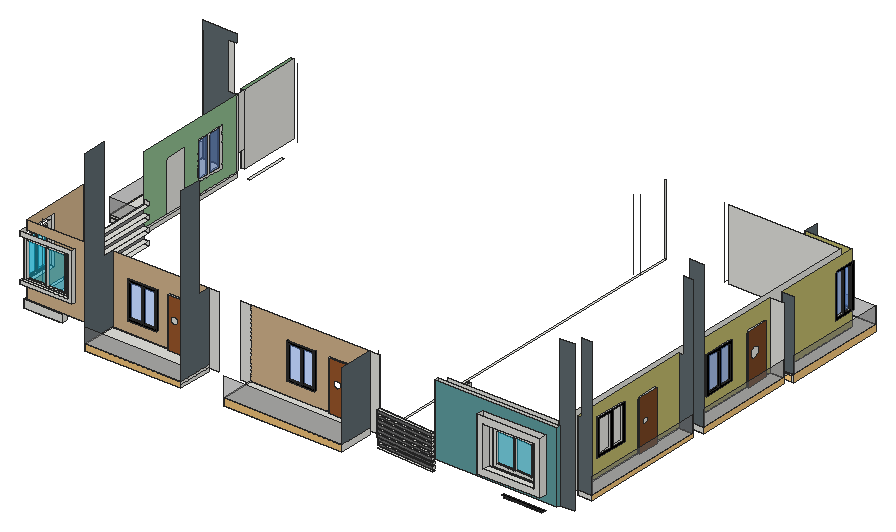
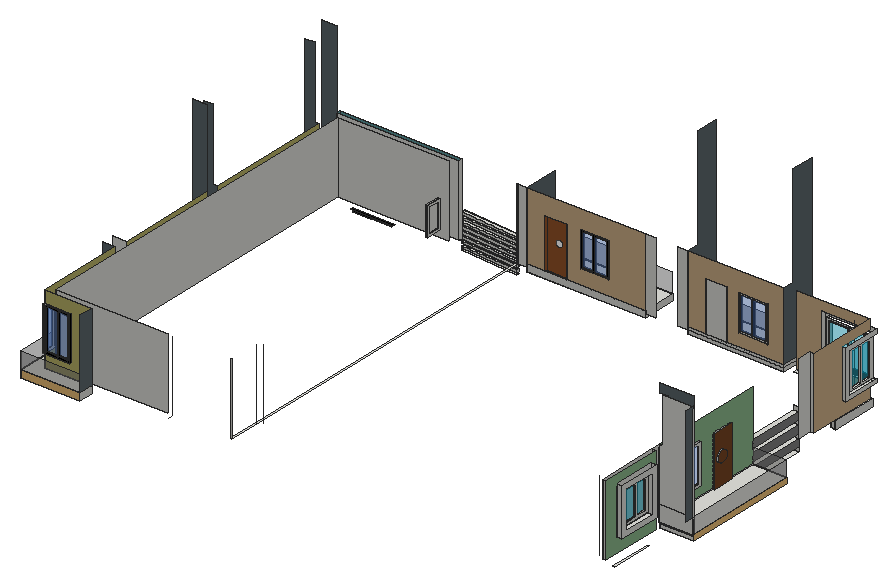
# SketchUp Ruby script. Lengths in inches.
U = 1.inch
M = Sketchup.active_model
def pt(a) = Geom::Point3d.new(a.map { |v| v * U })
def face(e, loops, mat)
  f = e.add_face(loops[0].map { |a| pt(a) })
  loops[1..].each { |l| e.add_face(l.map { |a| pt(a) }).erase! }
  f.material = f.back_material = mat if mat
  f
end
# faces: each face lists its corners as indices into pts; further lists are holes
def faces(e, pts, list, mat = nil) = list.each { |f| face(e, (f[0].is_a?(Array) ? f : [f]).map { |l| l.map { |i| pts[i] } }, mat) }
# xy, xz, yz: faces in a plane at the given z, y or x. An outline is a flat list of corners, or four numbers for a rectangle; further outlines are holes
def ring(l) = l.size == 4 ? [[l[0], l[1]], [l[2], l[1]], [l[2], l[3]], [l[0], l[3]]] : l.each_slice(2).to_a
def flat(e, list, mat, &to3) = list.each { |f| face(e, (f[0].is_a?(Array) ? f : [f]).map { |l| ring(l).map { |u, v| to3.(u, v) } }, mat) }
def xy(e, z, list, mat = nil) = flat(e, list, mat) { |x, y| [x, y, z] }
def xz(e, y, list, mat = nil) = flat(e, list, mat) { |x, z| [x, y, z] }
def yz(e, x, list, mat = nil) = flat(e, list, mat) { |y, z| [x, y, z] }
def lines(e, pts, list) = list.each { |a, b| e.add_line(pt(pts[a]), pt(pts[b])) }
# prism: a flat outline (further loops are holes) pulled along v
def prism(e, loops, v, mat = nil)
  f = face(e, loops, mat); d = Geom::Vector3d.new(v.map { |x| x * U })
  f.pushpull(f.normal.samedirection?(d) ? d.length : -d.length)
end
def box(e, o, s, mat = nil) = prism(e, [[o, [o[0] + s[0], o[1], o[2]], [o[0] + s[0], o[1] + s[1], o[2]], [o[0], o[1] + s[1], o[2]]]], [0, 0, s[2]], mat)
def at(x, y, z, deg = 0) = Geom::Transformation.translation(pt([x, y, z])) * Geom::Transformation.rotation(ORIGIN, Z_AXIS, deg.degrees)
def axes(o, x, y, z) = Geom::Transformation.new([*x, 0, *y, 0, *z, 0, *pt(o).to_a, 1])
def part(name) = M.definitions.add(name)
# library, detail: a bought-in or finely detailed component or shape, given as its bounding box
def library(name, o, s) = part(name).tap { |d| box(d.entities, o, s) }
def detail(e, o, s) = box(e.add_group.entities, o, s)
def put(e, d, t, mat = nil) = e.add_instance(d, t).tap { |i| i.material = mat if mat }
def group(e, t, mat = nil) = e.add_group.tap { |g| g.transformation = t; g.material = mat if mat }.entities
root = M.entities
M.materials.add("[0035_Tan]").color = [210, 180, 140]
M.materials.add("[0057_DarkKhaki]").color = [189, 183, 107]
M.materials.add("[0072_DarkSeaGreen]").color = [143, 188, 143]
M.materials.add("[0081_CadetBlue]").color = [95, 158, 160]
M.materials.add("[0133_Gray]").color = [128, 128, 128]
M.materials.add("[0134_DimGray]").color = [105, 105, 105]
M.materials.add("[0137_Black]").color = [0, 0, 0]
M.materials.add("[Formica Speckled Grey]").color = [94, 105, 111]
M.materials.add("[Translucent Glass Blue]").color = [100, 149, 237]
M.materials["[Translucent Glass Blue]"].alpha = 0.5
M.materials.add("[Translucent Glass Gray]").color = [128, 128, 128]
M.materials["[Translucent Glass Gray]"].alpha = 0.5
M.materials.add("[Translucent Glass Tinted]").color = [8, 201, 241]
M.materials["[Translucent Glass Tinted]"].alpha = 0.48
M.materials.add("[Wood Cherry Original]").color = [152, 86, 42]
M.materials.add("[Wood OSB]").color = [240, 195, 122]
M.materials.add("[Wood Veneer 01]").color = [120, 70, 37]
xy(root,471.13,[[972.47,731.11,975.47,770.48]])
xy(root,471.13,[[931.65,770.48,972.47,773.48],[972.47,770.48,975.47,773.48]],"[0137_Black]")
xy(root,471.63,[[80.8125,615.71,83.8125,687.27]])
xy(root,472.53,[[912.27,155.58,914.48,158.58]])
xy(root,472.53,[[880.02,155.58,912.27,158.58],[914.48,155.58,944.52,158.58]],"[0137_Black]")
xy(root,472.62,[[83.8125,295.24,92.8125,392.06]])
xy(root,474.43,[[766.19,148.96,766.41,152.52,668.06,158.52,667.84,154.96]])
xy(root,474.85,[[86.8125,155.58,108.25,158.58],[109.36,155.58,129.6875,158.58],[86.8125,158.58,108.25,158.77],[109.36,158.58,129.6875,158.77],[80.8125,161.58,83.8125,184.96],
  [80.8125,186.77,83.8125,211.96]])
xy(root,475.53,[[877.02,155.58,947.52,158.58]],"[0137_Black]")
xy(root,477.48,[[766.19,148.96,667.84,154.96,668.06,158.52,766.41,152.52]])
xy(root,477.85,[[80.8125,155.58,83.8125,158.77],[83.8125,155.58,132.6875,158.58],[83.8125,158.58,132.6875,158.77],[80.8125,158.77,83.8125,214.96]])
xy(root,479.56,[[74.8125,149.58,74.8125,227.52,83.8125,227.52,83.8125,158.58,140.48,158.58,140.48,149.58]])
xy(root,480.06,[[83.8125,295.24,92.8125,392.06]])
xy(root,481.68,[[766.19,148.96,766.41,152.52,668.06,158.52,667.84,154.96]])
xy(root,482.83,[[975.47,621.6875,975.47,770.48,896.3125,770.48,896.3125,794.48,996.47,794.48,996.47,621.6875]],"[Wood OSB]")
xy(root,484.73,[[766.19,148.96,667.84,154.96,668.06,158.52,766.41,152.52]])
xy(root,485.43,[[450.92,100.8,651.23,158.58]],"[Wood OSB]")
xy(root,486.18,[[217.79,100.8,379.72,158.58],[26.03,392.06,83.8125,587.65]],"[Wood OSB]")
xy(root,488.93,[[766.19,148.96,766.41,152.52,668.06,158.52,667.84,154.96]])
xy(root,489.56,[[972.47,431.23,996.47,600.85]],"[Wood OSB]")
xy(root,491.98,[[766.05,146.53,667.69,152.53,668.06,158.52,766.41,152.52]])
xy(root,492.18,[[74.8125,149.58,140.48,149.58,140.48,152.58,77.8125,152.58,77.8125,227.52,74.8125,227.52],[77.8125,152.58,83.8125,158.58],[83.8125,152.58,140.48,158.58],[140.48,152.58,200.97,158.58],[765.79,152.58,766.41,158.58],
  [766.41,152.58,972.47,158.58],[77.8125,158.58,83.8125,227.52],[666.68,158.58,668.06,709.05],[77.8125,227.52,83.8125,271.7],[77.8125,604.3125,83.8125,709.05],
  [666.68,709.05,668.06,761.48]])
xy(root,492.18,[[972.47,194.93,996.47,408.53]],"[Wood OSB]")
xy(root,492.56,[[83.8125,295.24,92.8125,392.06]])
xy(root,494.83,[[975.47,621.6875,996.47,621.6875,996.47,794.48,896.3125,794.48,896.3125,770.48,975.47,770.48]])
xy(root,496.06,[[26.03,392.06,83.8125,392.06,83.8125,440.49,80.8125,440.49,80.8125,476.49,83.8125,476.49,83.8125,587.65,26.03,587.65],[80.8125,440.49,83.8125,476.49],[26.03,587.65,83.8125,589.72]])
xy(root,496.18,[[766.05,146.53,766.41,152.52,668.06,158.52,667.69,152.53]])
xy(root,496.47,[[217.79,100.8,379.72,100.8,379.72,158.58,349.74,158.58,349.74,155.58,313.74,155.58,313.74,158.58,217.79,158.58],[450.92,100.8,651.23,100.8,651.23,158.58,620.77,158.58,620.77,155.58,584.77,155.58,584.77,158.58,450.92,158.58],[313.74,155.58,349.74,158.58],[584.77,155.58,620.77,158.58]])
xy(root,498.56,[[972.47,431.23,996.47,431.23,996.47,600.85,972.47,600.85,972.47,588.41,975.47,588.41,975.47,552.41,972.47,552.41],[972.47,552.41,975.47,588.41]])
xy(root,499.19,[[972.47,194.93,996.47,194.93,996.47,408.53,972.47,408.53,972.47,358.375,975.47,358.375,975.47,322.375,972.47,322.375],[972.47,322.375,975.47,358.375]])
xy(root,499.23,[[766.05,146.53,667.69,152.53,668.06,158.52,766.41,152.52]])
xy(root,500,[[83.8125,295.24,92.8125,392.06]])
xy(root,503.43,[[766.05,146.53,766.41,152.52,668.06,158.52,667.69,152.53]])
xy(root,503.75,[[846.5,140.58,952.45,152.58]])
xy(root,506.48,[[766.05,146.53,667.69,152.53,668.06,158.52,766.41,152.52]])
xy(root,510.68,[[766.05,146.53,766.41,152.52,668.06,158.52,667.69,152.53]])
xy(root,512.5,[[83.8125,295.24,92.8125,392.06]])
xy(root,513.73,[[766.05,146.53,667.69,152.53,668.06,158.52,766.41,152.52]])
xy(root,514.41,[[857.16,140.58,941.79,152.58]])
xy(root,514.48,[[80.8125,505.73,83.8125,555.41]])
xy(root,515.54,[[71.8125,146.58,71.8125,211.02,77.8125,211.02,77.8125,152.58,159.375,152.58,159.375,146.58]])
xy(root,517.48,[[80.8125,508.73,83.8125,527.36],[80.8125,530.57,83.8125,552.41]])
xy(root,517.58,[[245.3125,155.58,294.5,158.58]])
xy(root,517.93,[[766.05,146.53,766.41,152.52,668.06,158.52,667.69,152.53]])
xy(root,518.04,[[68.8125,613.85,77.8125,685.91]])
xy(root,518.4,[[866.65,149.58,936.8125,152.58]])
xy(root,518.53,[[930.09,770.48,972.47,773.48]])
xy(root,518.59,[[972.47,735.61,975.47,770.48],[972.47,770.48,975.47,773.48]])
xy(root,519.94,[[83.8125,295.24,92.8125,392.06]])
xy(root,520.39,[[514.1,155.58,560.92,158.58]],"[0137_Black]")
xy(root,520.58,[[248.3125,155.58,269.91,158.58],[272.57,155.58,291.5,158.58]],"[0137_Black]")
xy(root,520.98,[[766.05,146.53,667.69,152.53,668.06,158.52,766.41,152.52]])
xy(root,521.53,[[933.09,770.48,948.82,773.48],[951.28,770.48,969.47,773.48]],"[0137_Black]")
xy(root,521.54,[[71.8125,146.58,151.54,146.58,151.54,152.58,77.8125,152.58,77.8125,203.77,71.8125,203.77]])
xy(root,521.59,[[972.47,738.61,975.47,753.05],[972.47,755.68,975.47,767.48]],"[0137_Black]")
xy(root,522.6,[[74.8125,149.58,147.9375,152.58],[74.8125,152.58,77.8125,197.89]])
xy(root,523.39,[[517.1,155.58,537.51,158.58],[540.34,155.58,557.92,158.58]],"[0137_Black]")
xy(root,523.48,[[972.47,464.5,975.47,516.9375]])
xy(root,523.95,[[872.2,149.58,901.73,152.58],[904.37,149.58,931.26,152.58]])
xy(root,525.18,[[766.05,146.53,766.41,152.52,668.06,158.52,667.69,152.53]])
xy(root,525.6,[[80.8125,149.58,112.875,152.58],[114.7,149.58,144.9375,152.58],[74.8125,155.58,77.8125,172.52],[74.8125,175.24,77.8125,194.89]])
xy(root,525.84,[[68.8125,621.65,77.8125,678.11]])
xy(root,526.48,[[972.47,467.5,975.47,490.72],[972.47,493.16,975.47,513.9375]],"[0137_Black]")
xy(root,527.53,[[763.41,201.89,766.41,227.45]])
xy(root,528.23,[[766.05,146.53,667.69,152.53,668.06,158.52,766.41,152.52]])
xy(root,529.02,[[74.8125,624.83,77.8125,674.93]])
xy(root,530.53,[[763.41,204.89,766.41,224.45]])
xy(root,531.54,[[972.47,234.17,975.47,290.11]])
xy(root,532.35,[[74.8125,628.16,77.8125,647],[74.8125,649.88,77.8125,671.6]])
xy(root,532.43,[[766.05,146.53,766.41,152.52,668.06,158.52,667.69,152.53],[83.8125,295.24,92.8125,392.06]])
xy(root,572.16,[[763.41,204.89,766.41,224.45]])
xy(root,575.16,[[763.41,201.89,766.41,227.45]])
xz(root,100.8,[[217.79,496.47,379.72,522.05],[450.92,496.47,651.23,529.78]],"[Translucent Glass Gray]")
xz(root,100.8,[[450.92,485.43,651.23,496.47],[217.79,486.18,379.72,496.47]],"[Wood OSB]")
xz(root,140.58,[[[846.5,503.75,952.45,593.76],[857.16,514.41,941.79,583.1]]])
xz(root,146.58,[[71.8125,515.54,159.375,515.54,159.375,596.48,71.8125,596.48,71.8125,588.98,151.54,588.98,151.54,521.54,71.8125,521.54]])
xz(root,149.58,[[74.8125,479.56,140.48,492.18],[[866.65,518.4,936.8125,579.13],[872.2,523.95,901.73,573.58],[904.37,523.95,931.26,573.58]],[[74.8125,522.6,147.9375,586.79],[80.8125,525.6,112.875,583.79],[114.7,525.6,144.9375,583.79]]])
xz(root,152.58,[[[846.5,503.75,952.45,593.76],[857.16,514.41,941.79,583.1]],[[857.16,514.41,941.79,583.1],[866.65,518.4,936.8125,579.13]],[[866.65,518.4,936.8125,579.13],[872.2,523.95,901.73,573.58],[904.37,523.95,931.26,573.58]],[77.8125,521.54,151.54,521.54,151.54,588.98,77.8125,588.98,77.8125,586.79,147.9375,586.79,147.9375,522.6,77.8125,522.6]])
xz(root,152.58,[[77.8125,492.18,200.97,492.18,200.97,612.18,77.8125,612.18,77.8125,596.48,159.375,596.48,159.375,515.54,77.8125,515.54]],"[0035_Tan]")
xz(root,152.58,[[[766.41,492.18,972.47,612.18],[846.5,503.75,952.45,593.76]]],"[0081_CadetBlue]")
xz(root,152.58,[[872.2,523.95,901.73,573.58],[904.37,523.95,931.26,573.58],[80.8125,525.6,112.875,583.79],[114.7,525.6,144.9375,583.79]],"[Translucent Glass Tinted]")
xz(root,155.58,[[74.8125,525.6,77.8125,583.79]])
xz(root,155.58,[[[245.3125,517.58,294.5,579.7],[248.3125,520.58,269.91,576.7],[272.57,520.58,291.5,576.7]],[[514.1,520.39,560.92,580.89],[517.1,523.39,537.51,577.89],[540.34,523.39,557.92,577.89]]],"[0137_Black]")
xz(root,155.58,[[[313.74,496.47,349.74,580.47],[323.72,538.36,322.125,538.6875,320.67,539.43,319.45,540.51,318.5625,541.88,318.05,543.43,317.96,545.06,318.29,546.65,319.03,548.11,320.12,549.33,321.48,550.22,323.03,550.73,324.66,550.82,326.26,550.49,327.72,549.75,328.93,548.66,329.82,547.3,330.33,545.75,330.43,544.12,330.09,542.52,329.36,541.07,328.27,539.85,326.9,538.96,325.35,538.45]],[[584.77,496.47,620.77,580.47],[599.13,537.91,597.53,538.12,596.04,538.73,594.75,539.72,593.77,541,593.15,542.49,592.94,544.09,593.15,545.69,593.77,547.1875,594.75,548.47,596.04,549.45,597.53,550.07,599.13,550.28,600.73,550.07,602.22,549.45,603.5,548.47,604.49,547.1875,605.11,545.69,605.32,544.09,605.11,542.49,604.49,541,603.5,539.72,602.22,538.73,600.73,538.12]]],"[Wood Cherry Original]")
xz(root,158.58,[[83.8125,479.56,140.48,492.18],[450.92,485.43,651.23,496.47],[217.79,486.18,379.72,492.18],[217.79,492.18,379.72,496.47],[379.72,492.18,396.54,612.18],
  [434.03,492.18,450.85,612.18],[651.23,492.18,666.68,612.18],[666.68,492.18,668.06,612.18],[766.41,492.18,972.47,612.18],[313.74,496.47,349.74,580.47],
  [[245.3125,517.58,294.5,579.7],[248.3125,520.58,269.91,576.7],[272.57,520.58,291.5,576.7]]])
xz(root,158.58,[[[450.85,492.18,450.92,492.18,450.92,496.47,584.77,496.47,584.77,580.47,620.77,580.47,620.77,496.47,651.23,496.47,651.23,612.18,450.85,612.18],[514.1,520.39,560.92,580.89]],[[217.79,496.47,313.74,496.47,313.74,580.47,349.74,580.47,349.74,496.47,379.72,496.47,379.72,612.18,217.79,612.18],[245.3125,517.58,294.5,579.7]]],"[0035_Tan]")
xz(root,158.58,[[972.47,492.18,996.47,744.18]],"[Formica Speckled Grey]")
xz(root,158.58,[[248.3125,520.58,269.91,576.7],[272.57,520.58,291.5,576.7],[517.1,523.39,537.51,577.89],[540.34,523.39,557.92,577.89]],"[Translucent Glass Blue]")
xz(root,167.58,[[775.41,492.18,963.47,612.18]])
xz(root,172.52,[[74.8125,525.6,77.8125,583.79]])
xz(root,175.24,[[74.8125,525.6,77.8125,583.79]])
xz(root,194.89,[[74.8125,525.6,77.8125,583.79]])
xz(root,194.93,[[972.47,492.18,996.47,499.19]])
xz(root,194.93,[[972.47,499.19,972.47,612.18,980.72,612.18,980.72,732.18,996.47,732.18,996.47,499.19]],"[Formica Speckled Grey]")
xz(root,197.89,[[74.8125,522.6,77.8125,586.79]])
xz(root,201.89,[[763.41,527.53,766.41,575.16]])
xz(root,203.77,[[71.8125,521.36,77.8125,521.54],[71.8125,521.54,77.8125,588.98]])
xz(root,204.89,[[763.41,530.53,766.41,572.16]])
xz(root,211.02,[[71.8125,515.54,77.8125,596.48]])
xz(root,224.45,[[763.41,530.53,766.41,572.16]])
xz(root,227.45,[[763.41,527.53,766.41,575.16]])
xz(root,227.52,[[74.8125,479.56,77.8125,492.18],[77.8125,479.56,83.8125,492.18]])
xz(root,234.17,[[972.47,531.54,975.47,592.54]],"[0137_Black]")
xz(root,271.7,[[77.8125,492.18,83.8125,612.18]])
xz(root,290.11,[[972.47,531.54,975.47,592.54]],"[0137_Black]")
xz(root,295.24,[[83.8125,472.62,92.8125,480.06],[83.8125,492.56,92.8125,500],[83.8125,512.5,92.8125,519.94],[83.8125,532.43,92.8125,539.88]])
xz(root,322.375,[[972.47,499.19,975.47,583.19]],"[Wood Veneer 01]")
xz(root,358.375,[[972.47,499.19,975.47,583.19]],"[Wood Veneer 01]")
xz(root,392.06,[[83.8125,472.62,92.8125,480.06],[26.03,486.18,83.8125,492.18],[26.03,492.18,83.8125,492.56],[26.03,492.56,83.8125,496.06],[83.8125,492.56,92.8125,500],
  [83.8125,512.5,92.8125,519.94],[83.8125,532.43,92.8125,539.88]])
xz(root,392.06,[[26.03,496.06,83.8125,522.85]],"[Translucent Glass Gray]")
xz(root,408.53,[[972.47,492.18,996.47,499.19]])
xz(root,408.53,[[972.47,499.19,996.47,499.19,996.47,732.18,981.03,732.18,981.03,612.18,972.47,612.18]],"[Formica Speckled Grey]")
xz(root,431.23,[[972.47,489.56,996.47,498.56]])
xz(root,431.23,[[972.47,498.56,996.47,744.18]],"[Formica Speckled Grey]")
xz(root,440.49,[[80.8125,496.06,83.8125,580.06]],"[Wood Veneer 01]")
xz(root,464.5,[[972.47,523.48,975.47,585.79]],"[0137_Black]")
xz(root,467.5,[[972.47,526.48,975.47,582.79]],"[0137_Black]")
xz(root,476.49,[[80.8125,496.06,83.8125,580.06]],"[Wood Veneer 01]")
xz(root,490.72,[[972.47,526.48,975.47,582.79]],"[0137_Black]")
xz(root,493.16,[[972.47,526.48,975.47,582.79]],"[0137_Black]")
xz(root,505.73,[[80.8125,514.48,83.8125,580.48]])
xz(root,508.73,[[80.8125,517.48,83.8125,577.48]])
xz(root,513.9375,[[972.47,526.48,975.47,582.79]],"[0137_Black]")
xz(root,516.9375,[[972.47,523.48,975.47,585.79]],"[0137_Black]")
xz(root,527.36,[[80.8125,517.48,83.8125,577.48]])
xz(root,530.57,[[80.8125,517.48,83.8125,577.48]])
xz(root,552.41,[[80.8125,517.48,83.8125,577.48]])
xz(root,552.41,[[972.47,498.56,975.47,582.56]],"[Wood Veneer 01]")
xz(root,555.41,[[80.8125,514.48,83.8125,580.48]])
xz(root,587.65,[[26.03,486.18,83.8125,492.18],[26.03,492.18,83.8125,496.06]])
xz(root,587.65,[[26.03,496.06,83.8125,496.06,83.8125,612.18,68.8125,612.18,68.8125,689.85,83.8125,689.85,83.8125,704.68,26.03,704.68]],"[Formica Speckled Grey]")
xz(root,588.41,[[972.47,498.56,975.47,582.56]],"[Wood Veneer 01]")
xz(root,589.72,[[26.03,496.06,83.8125,522.6],[26.03,522.6,83.8125,522.6,83.8125,612.18,77.8125,612.18,77.8125,689.85,26.03,689.85]])
xz(root,600.85,[[972.47,489.56,996.47,498.56],[972.47,498.56,996.47,612.18]])
xz(root,604.3125,[[77.8125,492.18,83.8125,522.6],[77.8125,522.6,83.8125,612.18]])
xz(root,613.85,[[68.8125,518.04,77.8125,597.29]])
xz(root,621.65,[[68.8125,525.84,77.8125,589.49]])
xz(root,621.6875,[[993.47,482.83,996.47,492.65],[975.47,492.65,993.47,494.83],[993.47,492.65,996.47,494.83]])
xz(root,621.6875,[[975.47,494.83,996.47,612.18]],"[Formica Speckled Grey]")
xz(root,624.83,[[74.8125,529.02,77.8125,586.31]])
xz(root,628.16,[[74.8125,532.35,77.8125,582.97]])
xz(root,647,[[74.8125,532.35,77.8125,582.97]])
xz(root,649.88,[[74.8125,532.35,77.8125,582.97]])
xz(root,671.6,[[74.8125,532.35,77.8125,582.97]])
xz(root,674.93,[[74.8125,529.02,77.8125,586.31]])
xz(root,678.11,[[68.8125,525.84,77.8125,589.49]])
xz(root,685.91,[[68.8125,518.04,77.8125,597.29]])
xz(root,709.05,[[77.8125,492.18,83.8125,612.18]])
xz(root,735.61,[[972.47,518.59,975.47,592.47]])
xz(root,738.61,[[972.47,521.59,975.47,589.47]],"[0137_Black]")
xz(root,753.05,[[972.47,521.59,975.47,589.47]],"[0137_Black]")
xz(root,755.68,[[972.47,521.59,975.47,589.47]],"[0137_Black]")
xz(root,761.48,[[666.68,492.18,668.06,612.18],[775.41,492.18,963.47,612.18]])
xz(root,767.48,[[972.47,521.59,975.47,589.47]],"[0137_Black]")
xz(root,770.48,[[896.3125,482.83,918.4,494.83],[918.4,482.83,975.47,494.83],[[930.09,518.53,972.47,592.47],[951.28,521.53,969.47,589.47],[933.09,521.53,948.82,589.47]],[972.47,518.53,975.47,518.59],[972.47,518.59,975.47,592.47]])
xz(root,770.48,[[896.3125,494.83,896.3125,612.18,975.47,612.18,975.47,592.47,930.09,592.47,930.09,518.53,975.47,518.53,975.47,494.83]],"[0057_DarkKhaki]")
xz(root,770.48,[[933.09,521.53,948.82,589.47],[951.28,521.53,969.47,589.47]],"[Translucent Glass Blue]")
xz(root,773.48,[[[930.09,518.53,972.47,592.47],[951.28,521.53,969.47,589.47],[933.09,521.53,948.82,589.47]],[972.47,518.59,975.47,592.47]],"[0137_Black]")
xz(root,794.48,[[896.3125,494.83,996.47,523.26]],"[Translucent Glass Gray]")
xz(root,794.48,[[896.3125,482.83,996.47,494.83]],"[Wood OSB]")
yz(root,26.03,[[587.65,496.06,589.72,522.6],[587.65,522.6,589.72,689.85]])
yz(root,26.03,[[589.72,522.6,604.3125,689.85]],"[Formica Speckled Grey]")
yz(root,26.03,[[392.06,496.06,587.65,522.6]],"[Translucent Glass Gray]")
yz(root,26.03,[[392.06,486.18,587.65,496.06]],"[Wood OSB]")
yz(root,68.8125,[[[613.85,518.04,685.91,597.29],[621.65,525.84,678.11,589.49]]])
yz(root,71.8125,[[146.58,515.54,146.58,521.54,203.77,521.54,203.77,588.98,146.58,588.98,146.58,596.48,211.02,596.48,211.02,515.54]])
yz(root,74.8125,[[149.58,479.56,227.52,492.18],[[149.58,522.6,197.89,586.79],[175.24,525.6,194.89,583.79],[155.58,525.6,172.52,583.79]],[[624.83,529.02,674.93,586.31],[649.88,532.35,671.6,582.97],[628.16,532.35,647,582.97]]])
yz(root,77.8125,[[152.58,513.29,152.64,515.54],[152.58,515.54,152.64,521.36],[[613.85,518.04,685.91,597.29],[621.65,525.84,678.11,589.49]],[152.58,521.36,152.64,521.54],[152.64,521.36,203.77,521.54],
  [152.58,521.54,152.58,522.6,197.89,522.6,197.89,586.79,152.58,586.79,152.58,588.98,203.77,588.98,203.77,521.54],[[621.65,525.84,678.11,589.49],[624.83,529.02,674.93,586.31]],[[624.83,529.02,674.93,586.31],[649.88,532.35,671.6,582.97],[628.16,532.35,647,582.97]]])
yz(root,77.8125,[[152.58,492.18,152.58,513.29,152.64,513.29,152.64,515.54,211.02,515.54,211.02,596.48,152.58,596.48,152.58,612.18,271.7,612.18,271.7,492.18]],"[0035_Tan]")
yz(root,77.8125,[[[604.3125,492.18,709.05,612.18],[613.85,518.04,685.91,597.29]]],"[0072_DarkSeaGreen]")
yz(root,77.8125,[[155.58,525.6,172.52,583.79],[175.24,525.6,194.89,583.79],[628.16,532.35,647,582.97],[649.88,532.35,671.6,582.97]],"[Translucent Glass Tinted]")
yz(root,77.8125,[[462.9,532.38,460.57,532.68,458.4,533.58,456.54,535.01,455.11,536.88,454.21,539.05,453.9,541.38,454.21,543.71,455.11,545.88,456.54,547.74,458.4,549.17,460.57,550.07,462.9,550.38,465.23,550.07,467.4,549.17,469.27,547.74,470.7,545.88,471.6,543.71,471.9,541.38,471.6,539.05,470.7,536.88,469.27,535.01,467.4,533.58,465.23,532.68]],"[Wood Veneer 01]")
yz(root,80.8125,[[[505.73,514.48,555.41,580.48],[530.57,517.48,552.41,577.48],[508.73,517.48,527.36,577.48]],[149.58,525.6,152.58,583.79],[462.9,532.38,465.23,532.68,467.4,533.58,469.27,535.01,470.7,536.88,471.6,539.05,471.9,541.38,471.6,543.71,470.7,545.88,469.27,547.74,467.4,549.17,465.23,550.07,462.9,550.38,460.57,550.07,458.4,549.17,456.54,547.74,455.11,545.88,454.21,543.71,453.9,541.38,454.21,539.05,455.11,536.88,456.54,535.01,458.4,533.58,460.57,532.68]])
yz(root,80.8125,[[[440.49,496.06,476.49,580.06],[462.9,532.38,465.23,532.68,467.4,533.58,469.27,535.01,470.7,536.88,471.6,539.05,471.9,541.38,471.6,543.71,470.7,545.88,469.27,547.74,467.4,549.17,465.23,550.07,462.9,550.38,460.57,550.07,458.4,549.17,456.54,547.74,455.11,545.88,454.21,543.71,453.9,541.38,454.21,539.05,455.11,536.88,456.54,535.01,458.4,533.58,460.57,532.68]]],"[Wood Veneer 01]")
yz(root,83.8125,[[158.58,479.56,227.52,492.18],[392.06,486.18,587.65,492.18],[271.7,492.18,295.24,612.18],[392.06,492.18,587.65,496.06],[604.3125,492.18,709.05,612.18],
  [440.49,496.06,476.49,580.06],[587.65,496.06,589.72,612.18],[[505.73,514.48,555.41,580.48],[530.57,517.48,552.41,577.48],[508.73,517.48,527.36,577.48]],[589.72,522.6,604.3125,612.18]])
yz(root,83.8125,[[[392.06,496.06,392.06,612.18,587.65,612.18,587.65,496.06,476.49,496.06,476.49,580.06,440.49,580.06,440.49,496.06],[505.73,514.48,555.41,580.48]]],"[0072_DarkSeaGreen]")
yz(root,83.8125,[[295.24,480.06,392.06,492.56],[295.24,500,392.06,512.5],[295.24,519.94,392.06,532.43]],"[0133_Gray]")
yz(root,83.8125,[[508.73,517.48,527.36,577.48],[530.57,517.48,552.41,577.48]],"[Translucent Glass Blue]")
yz(root,112.875,[[149.58,525.6,152.58,583.79]])
yz(root,114.7,[[149.58,525.6,152.58,583.79]])
yz(root,140.48,[[149.58,479.56,158.58,492.18]])
yz(root,144.9375,[[149.58,525.6,152.58,583.79]])
yz(root,147.9375,[[149.58,522.6,152.58,586.79]])
yz(root,151.54,[[146.58,521.54,152.58,588.98]])
yz(root,159.375,[[146.58,515.54,152.58,596.48]])
yz(root,217.79,[[100.8,486.18,158.58,492.18],[100.8,492.18,158.58,496.47]])
yz(root,217.79,[[100.8,496.47,158.58,496.47,158.58,612.18,140.58,612.18,140.58,784.18,100.8,784.18]],"[Formica Speckled Grey]")
yz(root,245.3125,[[155.58,517.58,158.58,579.7]],"[0137_Black]")
yz(root,248.3125,[[155.58,520.58,158.58,576.7]],"[0137_Black]")
yz(root,269.91,[[155.58,520.58,158.58,576.7]],"[0137_Black]")
yz(root,272.57,[[155.58,520.58,158.58,576.7]],"[0137_Black]")
yz(root,291.5,[[155.58,520.58,158.58,576.7]],"[0137_Black]")
yz(root,294.5,[[155.58,517.58,158.58,579.7]],"[0137_Black]")
yz(root,313.74,[[155.58,496.47,158.58,580.47]])
yz(root,349.74,[[155.58,496.47,158.58,580.47]])
yz(root,379.72,[[100.8,486.18,158.58,492.18],[100.8,492.18,158.58,496.47]])
yz(root,379.72,[[100.8,496.47,100.8,784.18,137.58,784.18,137.58,612.18,158.58,612.18,158.58,496.47]],"[Formica Speckled Grey]")
yz(root,450.92,[[100.8,485.43,158.58,496.47]])
yz(root,514.1,[[155.58,520.39,158.58,580.89]],"[0137_Black]")
yz(root,517.1,[[155.58,523.39,158.58,577.89]],"[0137_Black]")
yz(root,537.51,[[155.58,523.39,158.58,577.89]],"[0137_Black]")
yz(root,540.34,[[155.58,523.39,158.58,577.89]],"[0137_Black]")
yz(root,557.92,[[155.58,523.39,158.58,577.89]],"[0137_Black]")
yz(root,560.92,[[155.58,520.39,158.58,580.89]],"[0137_Black]")
yz(root,584.77,[[155.58,496.47,158.58,580.47]])
yz(root,620.77,[[155.58,496.47,158.58,580.47]],"[Wood Cherry Original]")
yz(root,651.23,[[100.8,485.43,158.58,496.47]])
yz(root,651.23,[[100.8,496.47,158.58,612.18]],"[Formica Speckled Grey]")
yz(root,763.41,[[[201.89,527.53,227.45,575.16],[204.89,530.53,224.45,572.16]]])
yz(root,766.41,[[152.52,492.18,152.58,612.18],[152.58,492.18,158.58,612.18],[[201.89,527.53,227.45,575.16],[204.89,530.53,224.45,572.16]],[204.89,530.53,224.45,572.16]])
yz(root,846.5,[[140.58,503.75,152.58,593.76]])
yz(root,857.16,[[140.58,514.41,152.58,583.1]])
yz(root,866.65,[[149.58,518.4,152.58,579.13]])
yz(root,872.2,[[149.58,523.95,152.58,573.58]])
yz(root,896.3125,[[770.48,482.83,794.48,494.83]])
yz(root,896.3125,[[770.48,494.83,794.48,612.18]],"[Formica Speckled Grey]")
yz(root,901.73,[[149.58,523.95,152.58,573.58]])
yz(root,904.37,[[149.58,523.95,152.58,573.58]])
yz(root,930.09,[[770.48,518.53,773.48,592.47]],"[0137_Black]")
yz(root,931.26,[[149.58,523.95,152.58,573.58]])
yz(root,933.09,[[770.48,521.53,773.48,589.47]],"[0137_Black]")
yz(root,936.8125,[[149.58,518.4,152.58,579.13]])
yz(root,941.79,[[140.58,514.41,152.58,583.1]])
yz(root,948.82,[[770.48,521.53,773.48,589.47]],"[0137_Black]")
yz(root,951.28,[[770.48,521.53,773.48,589.47]],"[0137_Black]")
yz(root,952.45,[[140.58,503.75,152.58,593.76]])
yz(root,963.47,[[167.58,492.18,761.48,612.18]])
yz(root,969.47,[[770.48,521.53,773.48,589.47]],"[0137_Black]")
yz(root,972.47,[[431.23,489.56,600.85,498.56],[194.93,492.18,408.53,499.19],[552.41,498.56,588.41,582.56],[322.375,499.19,358.375,583.19],[770.48,518.53,773.48,518.59],
  [[735.61,518.59,770.48,592.47],[738.61,521.59,753.05,589.47],[755.68,521.59,767.48,589.47]],[770.48,518.59,773.48,592.47],[[234.17,531.54,290.11,592.54],[237.17,534.54,262.14,589.54],[266.68,534.54,287.11,589.54]]])
yz(root,972.47,[[[431.23,498.56,552.41,498.56,552.41,582.56,588.41,582.56,588.41,498.56,600.85,498.56,600.85,612.18,431.23,612.18],[464.5,523.48,516.9375,585.79]],[[194.93,499.19,322.375,499.19,322.375,583.19,358.375,583.19,358.375,499.19,408.53,499.19,408.53,612.18,194.93,612.18],[234.17,531.54,290.11,592.54]]],"[0057_DarkKhaki]")
yz(root,972.47,[[152.58,492.18,158.58,612.18]],"[0081_CadetBlue]")
yz(root,972.47,[[738.61,521.59,753.05,589.47],[755.68,521.59,767.48,589.47],[467.5,526.48,490.72,582.79],[493.16,526.48,513.9375,582.79]],"[Translucent Glass Blue]")
yz(root,975.47,[[621.6875,482.83,770.48,492.65],[621.6875,492.65,770.48,494.83]])
yz(root,975.47,[[621.6875,494.83,770.48,494.83,770.48,518.59,735.61,518.59,735.61,592.47,770.48,592.47,770.48,612.18,621.6875,612.18]],"[0057_DarkKhaki]")
yz(root,975.47,[[[735.61,518.59,770.48,592.47],[738.61,521.59,753.05,589.47],[755.68,521.59,767.48,589.47]],[770.48,518.59,773.48,592.47],[[464.5,523.48,516.9375,585.79],[467.5,526.48,490.72,582.79],[493.16,526.48,513.9375,582.79]],[[234.17,531.54,290.11,592.54],[237.17,534.54,262.14,589.54],[266.68,534.54,287.11,589.54]]],"[0137_Black]")
yz(root,975.47,[[[552.41,498.56,588.41,582.56],[565.29,537.46,562.96,537.77,560.79,538.67,558.93,540.1,557.5,541.96,556.6,544.13,556.29,546.46,556.6,548.79,557.5,550.96,558.93,552.83,560.79,554.26,562.96,555.16,565.29,555.46,567.62,555.16,569.79,554.26,571.65,552.83,573.08,550.96,573.98,548.79,574.29,546.46,573.98,544.13,573.08,541.96,571.65,540.1,569.79,538.67,567.62,537.77]],[[322.375,499.19,358.375,583.19],[334.56,539.19,333.22,539.37,331.97,539.89,330.89,540.71,330.07,541.79,329.55,543.04,329.37,544.38,329.55,545.72,330.07,546.97,330.89,548.05,331.97,548.875,333.22,549.39,334.56,549.57,335.9,549.39,337.15,548.875,338.23,548.05,339.05,546.97,339.57,545.72,339.75,544.38,339.57,543.04,339.05,541.79,338.23,540.71,337.15,539.89,335.9,539.37]]],"[Wood Veneer 01]")
yz(root,996.47,[[794.48,494.83,795,523.21]])
yz(root,996.47,[[621.6875,494.83,794.48,523.21],[431.23,498.56,600.85,526.28],[194.93,499.19,408.53,527.7]],"[Translucent Glass Gray]")
yz(root,996.47,[[621.6875,482.83,794.48,494.83],[431.23,489.56,600.85,498.56],[194.93,492.18,408.53,499.19]],"[Wood OSB]")
p = [[766.19,148.96,481.68],[667.84,154.96,481.68],[667.84,154.96,477.48],[766.19,148.96,477.48],[766.41,152.52,477.48],[766.41,152.52,481.68],
  [668.06,158.52,481.68],[668.06,158.52,477.48],[766.19,148.96,488.93],[667.84,154.96,488.93],[667.84,154.96,484.73],[766.19,148.96,484.73],
  [766.41,152.52,484.73],[766.41,152.52,488.93],[668.06,158.52,488.93],[668.06,158.52,484.73],[766.05,146.53,496.18],[667.69,152.53,496.18],
  [667.69,152.53,491.98],[766.05,146.53,491.98],[766.05,146.53,492.18],[766.41,152.52,491.98],[766.41,152.52,492.18],[668.06,158.52,496.18],
  [668.06,158.52,491.98],[766.41,152.52,496.18],[668.06,158.58,612.18],[668.06,158.58,492.18],[668.05,158.52,492.18],[668.05,158.52,612.18],
  [766.05,146.53,503.43],[667.69,152.53,503.43],[667.69,152.53,499.23],[766.05,146.53,499.23],[766.41,152.52,499.23],[766.41,152.52,503.43],
  [668.06,158.52,503.43],[668.06,158.52,499.23],[766.05,146.53,510.68],[667.69,152.53,510.68],[667.69,152.53,506.48],[766.05,146.53,506.48],
  [766.41,152.52,506.48],[766.41,152.52,510.68],[668.06,158.52,510.68],[668.06,158.52,506.48],[766.05,146.53,517.93],[667.69,152.53,517.93],
  [667.69,152.53,513.73],[766.05,146.53,513.73],[766.41,152.52,513.73],[766.41,152.52,517.93],[668.06,158.52,517.93],[668.06,158.52,513.73],
  [766.05,146.53,525.18],[667.69,152.53,525.18],[667.69,152.53,520.98],[766.05,146.53,520.98],[766.41,152.52,520.98],[766.41,152.52,525.18],
  [668.06,158.52,525.18],[668.06,158.52,520.98],[766.05,146.53,532.43],[667.69,152.53,532.43],[667.69,152.53,528.23],[766.05,146.53,528.23],
  [766.41,152.52,528.23],[766.41,152.52,532.43],[668.06,158.52,532.43],[668.06,158.52,528.23],[80.8125,462.9,532.38],[80.8125,460.57,532.68],
  [77.8125,460.57,532.68],[77.8125,462.9,532.38],[80.8125,465.23,532.68],[77.8125,465.23,532.68],[80.8125,458.4,533.58],[77.8125,458.4,533.58],
  [80.8125,467.4,533.58],[77.8125,467.4,533.58],[80.8125,456.54,535.01],[77.8125,456.54,535.01],[80.8125,469.27,535.01],[77.8125,469.27,535.01],
  [659.06,703.7,492.18],[659.06,703.7,612.18],[92.8125,703.7,492.18],[92.8125,703.7,612.18],[659.06,167.58,492.18],[659.06,167.58,612.18],
  [92.8125,167.58,492.18],[92.8125,167.58,612.18],[766.41,761.48,492.18],[766.41,770.48,492.18],[77.8125,152.64,521.36],[71.8125,152.64,521.36],
  [77.8125,152.58,521.36],[71.8125,152.58,521.36],[77.8125,158.58,485.06],[77.8125,158.58,492.18],[666.68,709.05,492.18],[666.68,709.05,612.18],
  [766.41,761.48,612.18],[975.47,770.48,492.65],[993.47,770.48,492.65]]
faces(root,p,[[0,1,2,3],[8,9,10,11],[16,17,18,19,20],[30,31,32,33],[38,39,40,41],[46,47,48,49],[54,55,56,57],[62,63,64,65]],"[0134_DimGray]")
faces(root,p,[[4,5,0,3],[6,5,4,7],[6,7,2,1],[12,13,8,11],[14,13,12,15],[14,15,10,9],[21,22,20,19],[23,24,18,17],
  [23,25,22,21,24],[22,25,16,20],[26,27,28,29],[34,35,30,33],[36,37,32,31],[36,35,34,37],[42,43,38,41],[44,45,40,39],
  [44,43,42,45],[50,51,46,49],[52,53,48,47],[52,51,50,53],[58,59,54,57],[60,61,56,55],[60,59,58,61],[66,67,62,65],
  [68,69,64,63],[68,67,66,69]])
faces(root,p,[[70,71,72,73],[74,70,73,75],[71,76,77,72],[78,74,75,79],[76,80,81,77],[82,78,79,83]],"[Wood Veneer 01]")
lines(root,p,[[84,85],[86,87],[88,89],[90,91],[92,93],[94,95],[96,97],[98,99],[100,101],[92,102],[103,104]])
